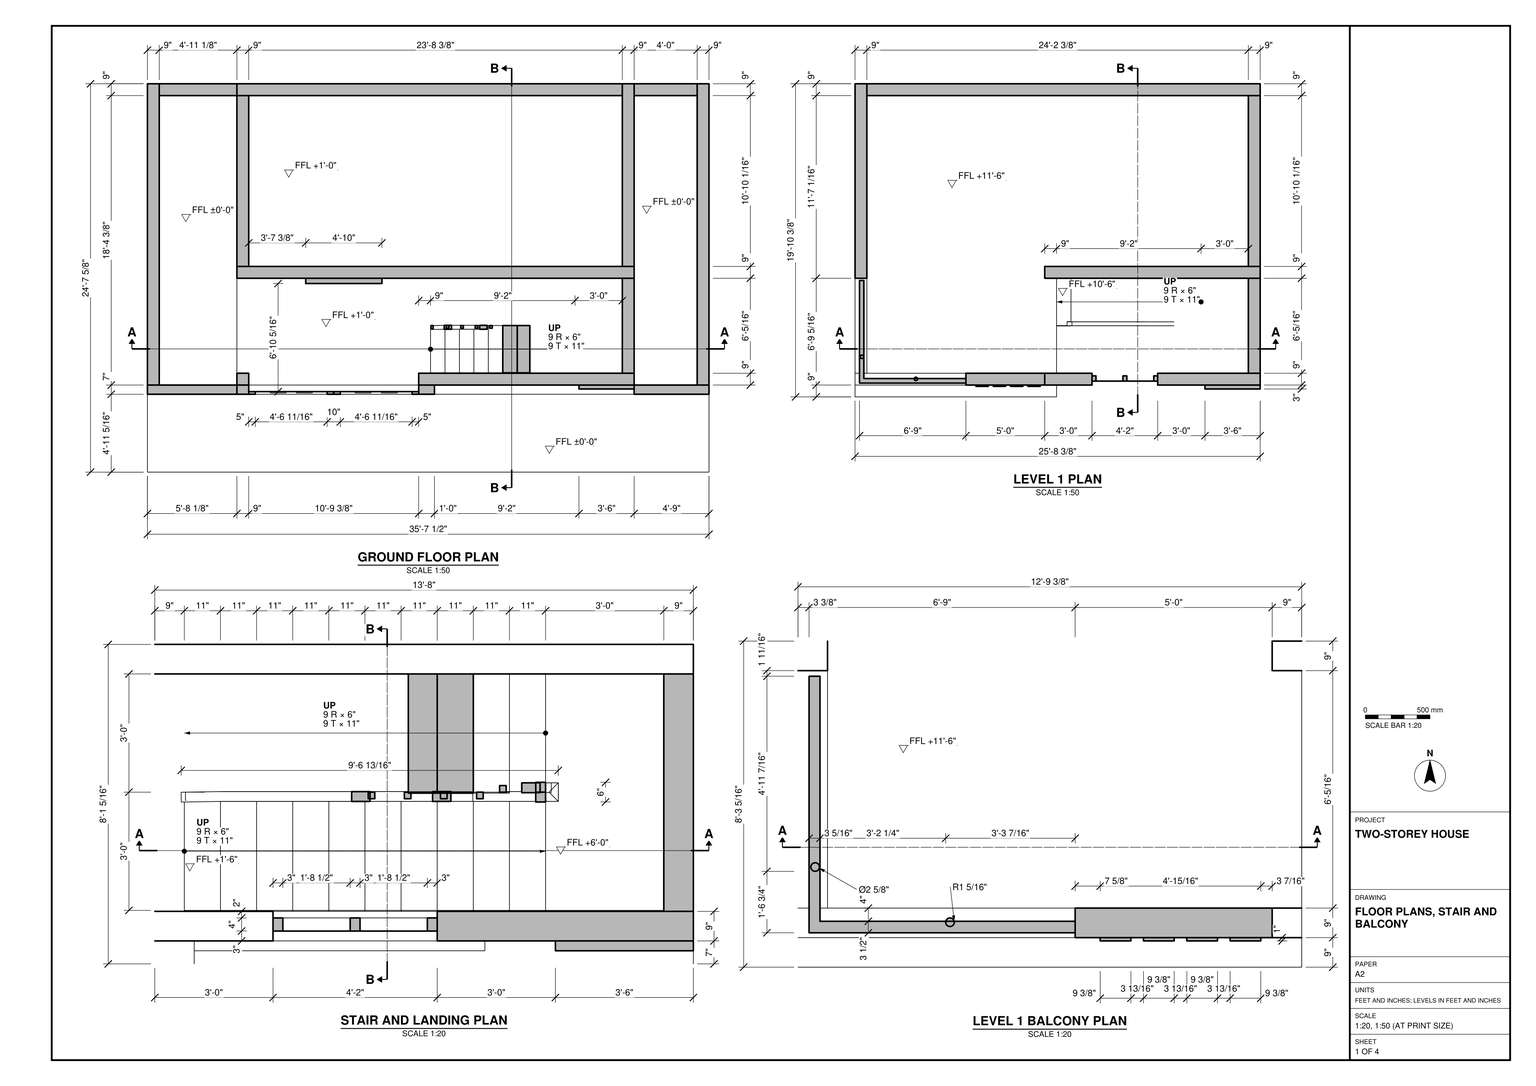
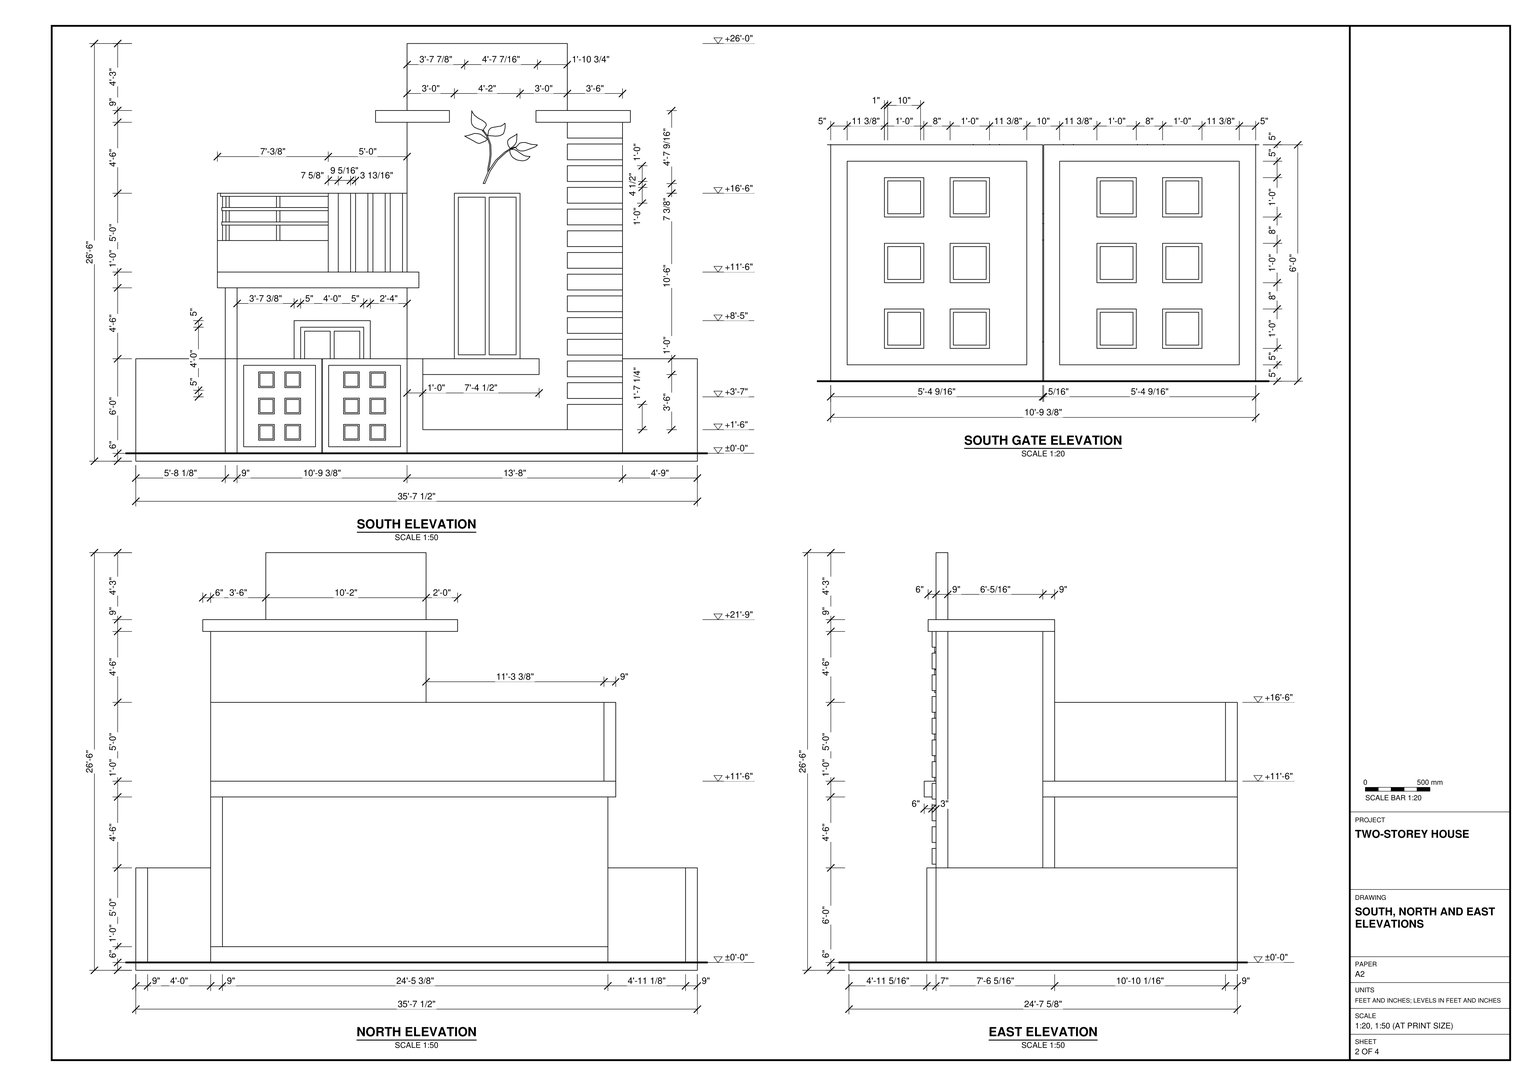
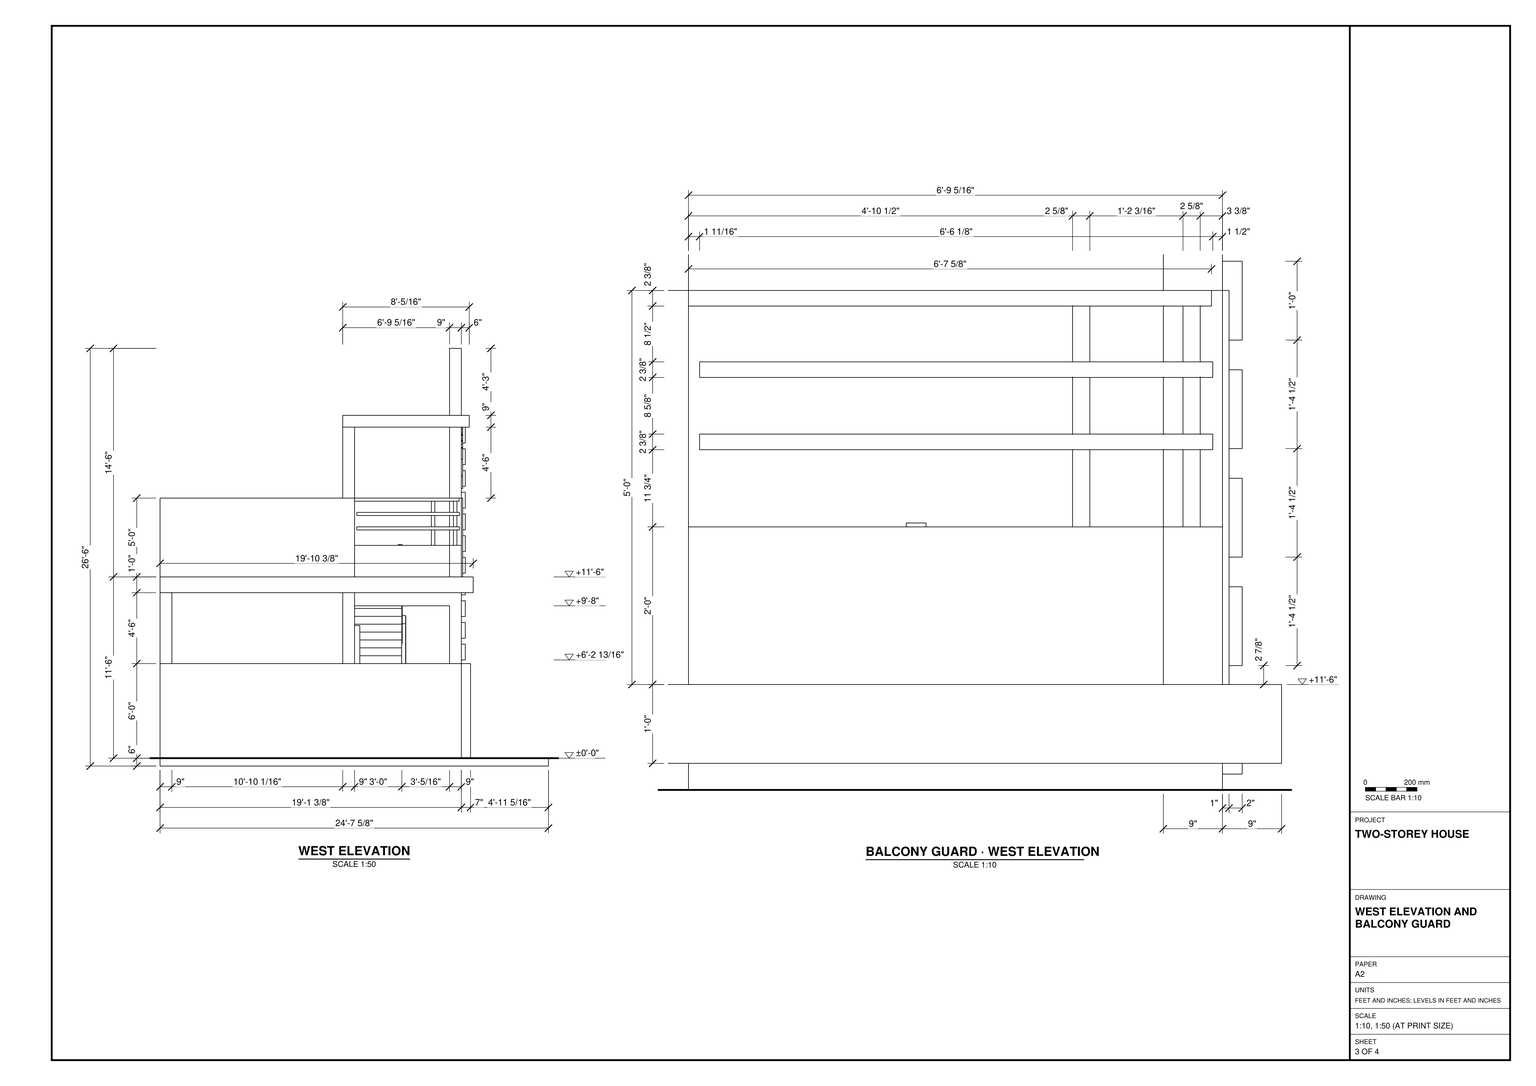
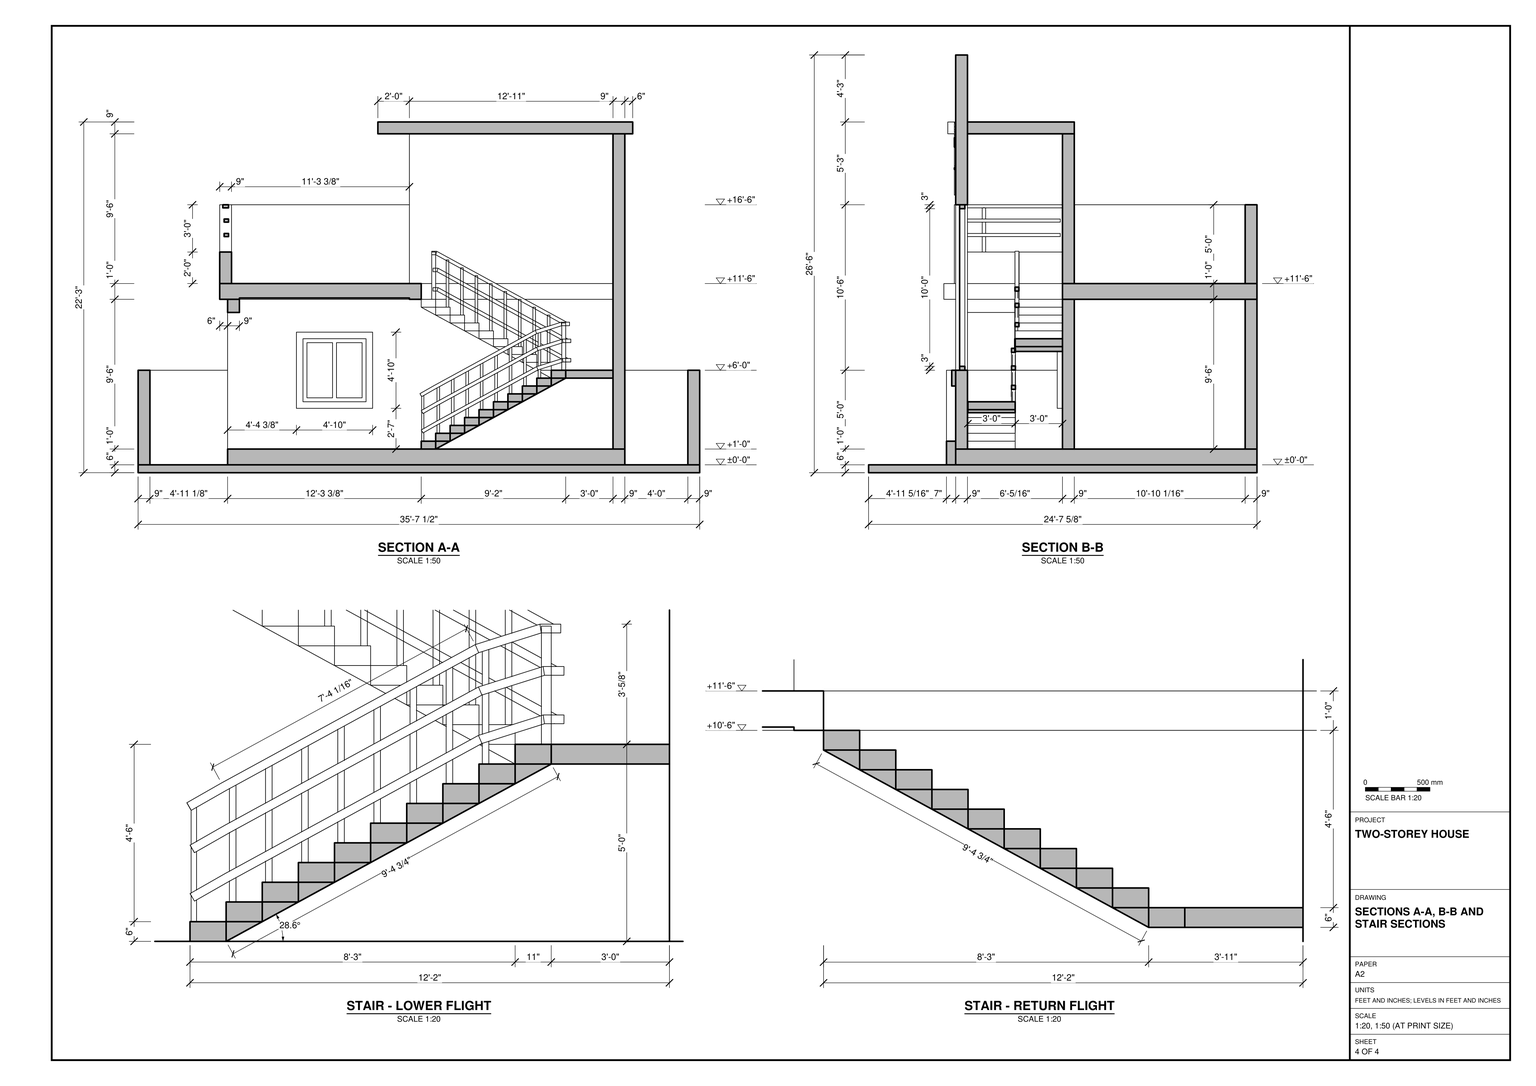
Build the two-storey house in SketchUp from task_files/diagram_01.pdf. Work in feet and inches. The overall model measures 35'-7 1/2" east to west, 24'-7 5/8" north to south and 26'-6" from the underside of the base to the highest wall. Use ±0'-0" as the ground-floor datum and +11'-6" as the Level 1 finished floor.

Start with the base slab, leaving the apron in front of the south gate and the narrow strips to either side of the house. Follow the ground-floor plan for the raised central floor, wall positions and 9" wall thicknesses where indicated. Model the paired gate leaves with their inset square panels and the framed opening behind the gate. Build the stair as two parallel flights that reverse direction at a common landing. Coordinate the stair opening in the upper slab with the flights below.

Use the elevations to distinguish the low terrace walls and balcony guard from the taller stair enclosure. Include the balcony slab edge, horizontal rails, uprights and adjoining vertical screen. Model the tall paired opening, projecting sill and horizontal bands on the south face of the stair enclosure, with the flat roof and raised wall above it. Decor and loose items shown may be represented by any suitable library component.

Keep shell elements such as walls, slabs and roof separate as groups or components. Group each furniture or joinery piece separately where shown, and use components for repeated parts. Save one SketchUp model as output_files/two_storey_house_with_a_return_stair_and_balcony.skp.

# SketchUp Ruby script. Lengths in inches.
U = 1.inch
M = Sketchup.active_model
def pt(a) = Geom::Point3d.new(a.map { |v| v * U })
def face(e, loops, mat)
  f = e.add_face(loops[0].map { |a| pt(a) })
  loops[1..].each { |l| e.add_face(l.map { |a| pt(a) }).erase! }
  f.material = f.back_material = mat if mat
  f
end
# faces: each face lists its corners as indices into pts; further lists are holes
def faces(e, pts, list, mat = nil) = list.each { |f| face(e, (f[0].is_a?(Array) ? f : [f]).map { |l| l.map { |i| pts[i] } }, mat) }
# xy, xz, yz: faces in a plane at the given z, y or x. An outline is a flat list of corners, or four numbers for a rectangle; further outlines are holes
def ring(l) = l.size == 4 ? [[l[0], l[1]], [l[2], l[1]], [l[2], l[3]], [l[0], l[3]]] : l.each_slice(2).to_a
def flat(e, list, mat, &to3) = list.each { |f| face(e, (f[0].is_a?(Array) ? f : [f]).map { |l| ring(l).map { |u, v| to3.(u, v) } }, mat) }
def xy(e, z, list, mat = nil) = flat(e, list, mat) { |x, y| [x, y, z] }
def xz(e, y, list, mat = nil) = flat(e, list, mat) { |x, z| [x, y, z] }
def yz(e, x, list, mat = nil) = flat(e, list, mat) { |y, z| [x, y, z] }
def lines(e, pts, list) = list.each { |a, b| e.add_line(pt(pts[a]), pt(pts[b])) }
# prism: a flat outline (further loops are holes) pulled along v
def prism(e, loops, v, mat = nil)
  f = face(e, loops, mat); d = Geom::Vector3d.new(v.map { |x| x * U })
  f.pushpull(f.normal.samedirection?(d) ? d.length : -d.length)
end
def box(e, o, s, mat = nil) = prism(e, [[o, [o[0] + s[0], o[1], o[2]], [o[0] + s[0], o[1] + s[1], o[2]], [o[0], o[1] + s[1], o[2]]]], [0, 0, s[2]], mat)
def at(x, y, z, deg = 0) = Geom::Transformation.translation(pt([x, y, z])) * Geom::Transformation.rotation(ORIGIN, Z_AXIS, deg.degrees)
def axes(o, x, y, z) = Geom::Transformation.new([*x, 0, *y, 0, *z, 0, *pt(o).to_a, 1])
def part(name) = M.definitions.add(name)
# library, detail: a bought-in or finely detailed component or shape, given as its bounding box
def library(name, o, s) = part(name).tap { |d| box(d.entities, o, s) }
def detail(e, o, s) = box(e.add_group.entities, o, s)
def put(e, d, t, mat = nil) = e.add_instance(d, t).tap { |i| i.material = mat if mat }
def group(e, t, mat = nil) = e.add_group.tap { |g| g.transformation = t; g.material = mat if mat }.entities
root = M.entities
M.materials.add("[Color M05]").color = [114, 114, 114]
M.materials.add("[Color M07]").color = [58, 58, 58]
M.materials.add("[Color M08]").color = [30, 30, 30]
M.materials.add("[Color M09]").color = [0, 0, 0]
M.materials.add("[Translucent Glass Gray]").color = [128, 128, 128]
M.materials["[Translucent Glass Gray]"].alpha = 0.5
c1 = part("Group\#4")
box(c1.entities,[0,0,0],[11,36,6])
c2 = part("Group\#5")
put(c2.entities,c1,at(22,0,12))
put(c2.entities,c1,at(11,0,6))
put(c2.entities,c1,at(44,0,24))
put(c2.entities,c1,at(33,0,18))
put(c2.entities,c1,at(0,0,0))
put(c2.entities,c1,at(55,0,30))
put(c2.entities,c1,at(99,0,54))
put(c2.entities,c1,at(66,0,36))
put(c2.entities,c1,at(77,0,42))
put(c2.entities,c1,at(88,0,48))
c3 = part("Group\#29")
box(c3.entities,[0,0,0],[3,3,36])
c4 = part("Group\#30")
xy(c4.entities,54.043,[[111.041,3.014,111.041,3.017,111.043,3.016]])
xy(c4.entities,56.716,[[111.723,3.695,113.885,5.858,111.723,5.858]])
yz(c4.entities,8.98,[[2.837,108.043,2.858,110.715,5.858,110.716,5.836,108.044]])
p = [[1.324,3.021,0],[1.361,0.022,0.021],[0.037,0,2.343],[0,2.999,2.321],[11.872,0.195,6.018],[10.57,0.173,8.352],
  [11.853,3.195,6.007],[10.552,3.173,8.341],[77.866,0.195,42.014],[88.886,0.195,48.025],[87.834,0.173,50.496],[76.586,0.173,44.36],
  [65.586,0.173,38.36],[54.586,0.173,32.36],[43.586,0.173,26.36],[32.586,0.173,20.36],[21.586,0.173,14.36],[22.866,0.195,12.014],
  [33.866,0.195,18.014],[44.866,0.195,24.014],[55.866,0.195,30.014],[66.866,0.195,36.014],[77.866,3.195,42.014],[88.886,3.195,48.025],
  [22.866,3.195,12.014],[33.866,3.195,18.014],[44.866,3.195,24.014],[55.866,3.195,30.014],[66.866,3.195,36.014],[76.586,3.173,44.36],
  [87.834,3.173,50.495],[21.586,3.173,14.36],[32.586,3.173,20.36],[43.586,3.173,26.36],[54.586,3.173,32.36],[65.586,3.173,38.36],
  [107.944,0.195,54.044],[107.532,0.173,56.716],[107.944,3.195,54.043],[107.532,3.173,56.715],[113.864,0.195,54.044],[113.885,0.173,56.716],
  [110.864,3.195,54.043],[111.041,3.017,54.043],[111.043,3.016,54.043],[113.864,5.836,54.044],[113.885,5.858,56.716],[100.095,2.837,60.014],
  [89.095,2.837,66.014],[78.095,2.837,72.014],[67.095,2.837,78.014],[56.095,2.837,84.014],[45.095,2.837,90.014],[34.095,2.837,96.014],
  [23.095,2.837,102.014],[12.041,2.837,108.043],[12.042,5.836,108.044],[23.095,5.836,102.014],[34.095,5.836,96.014],[45.095,5.836,90.014],
  [56.095,5.836,84.014],[67.095,5.836,78.014],[78.095,5.836,72.014],[89.095,5.836,66.014],[100.095,5.836,60.014],[111.042,5.836,54.044],
  [111.041,3.014,54.043],[111.041,2.837,54.043],[35.375,2.858,98.36],[24.375,2.858,104.36],[12.723,2.858,110.715],[111.723,2.858,56.715],
  [101.375,2.858,62.36],[90.375,2.858,68.36],[79.375,2.858,74.36],[68.375,2.858,80.36],[57.375,2.858,86.36],[46.375,2.858,92.36],
  [110.885,3.173,56.715],[12.723,5.858,110.716],[24.375,5.858,104.36],[35.375,5.858,98.36],[46.375,5.858,92.36],[57.375,5.858,86.36],
  [68.375,5.858,80.36],[79.375,5.858,74.36],[90.375,5.858,68.36],[101.375,5.858,62.36],[111.723,5.858,56.716],[111.043,3.016,56.715],
  [111.723,3.695,56.716],[8.98,2.837,108.043],[8.98,5.836,108.044],[8.98,2.858,110.715],[8.98,5.858,110.716]]
faces(c4.entities,p,[[0,1,2,3],[2,1,4,5],[1,0,6,4],[0,3,7,6],[3,2,5,7],[8,9,10,11,12,13,14,15,16,5,4,17,18,19,20,21],[22,23,9,8,21,20,19,18,17,4,6,24,25,26,27,28],[29,30,23,22,28,27,26,25,24,6,7,31,32,33,34,35],
  [11,10,30,29,35,34,33,32,31,7,5,16,15,14,13,12],[10,9,36,37],[9,23,38,36],[23,30,39,38],[30,10,37,39],[37,36,40,41],[36,38,42,43,44,40],[45,40,44],
  [41,40,45,46],[47,48,49,50,51,52,53,54,55,56,57,58,59,60,61,62,63,64,65,43,66,67],[68,69,70,55,54,53,52,51,50,49,48,47,67,71,72,73,74,75,76,77],[45,44,43,65],[38,39,78,42],[61,60,59,58,57,56,79,80,81,82,83,84,85,86,87,88,65,64,63,62],[46,45,65,88],[39,37,41,89,78],
  [41,46,90,89],[71,90,88,87,86,85,84,83,82,81,80,79,70,69,68,77,76,75,74,73,72],[56,55,91,92],[55,70,93,91],[79,56,92,94],[70,79,94,93]])
c5 = part("Group\#49")
box(c5.entities,[0,0,0],[42,3,12])
c6 = part("Group\#52")
box(c6.entities,[0,0,0],[9.34,1,60])
c7 = part("Group\#55")
prism(c7.entities,[[[82.03,5,0],[82.03,1.5,0],[1,1.5,0],[1,79.63,0],[4.34,79.63,0],[4.34,5,0]]],[0,0,2.375])
c8 = part("Group\#57")
prism(c8.entities,[[[0.38,2.24,0],[0.66,2.45,0],[0.97,2.58,0],[1.3125,2.625,0],[1.65,2.58,0],[1.97,2.45,0],[2.24,2.24,0],[2.45,1.97,0],[2.58,1.65,0],[2.625,1.3125,0],[2.58,0.97,0],[2.45,0.66,0],[2.24,0.38,0],[1.97,0.18,0],[1.65,0.04,0],[1.3125,0,0],[0.97,0.04,0],[0.66,0.18,0],[0.38,0.38,0],[0.18,0.66,0],[0.04,0.97,0],[0,1.3125,0],[0.04,1.65,0],[0.18,1.97,0]]],[0,0,33.75])
c9 = part("Group\#62")
prism(c9.entities,[[[12,0,0],[12,0,12],[0,0,12],[0,0,0]],[[11,0,11],[11,0,1],[1,0,1],[1,0,11]]],[0,1,0])
p = [[216,109.92,60],[226.51,110.09,66],[237.51,110.09,72],[248.51,110.09,78],[259.51,110.09,84],[270.51,110.09,90],
  [281.51,110.09,96],[292.51,110.09,102],[303.51,110.09,108],[322.51,110.09,114],[327.08,110.09,114],[327.08,113.09,114],
  [325.51,113.09,114],[314.51,113.09,120],[303.51,113.09,126],[292.51,113.09,132],[281.51,113.09,138],[270.51,113.09,144],
  [259.51,113.09,150],[248.51,113.09,156],[237.51,113.09,162],[226.51,113.09,168],[223.51,113.09,168],[215.51,66.29,132],
  [215.51,66.29,144],[206.51,66.29,132],[206.51,66.29,258],[238.78,66.29,258],[238.78,66.29,267],[206.51,66.29,267],
  [328.51,66.29,267],[304.64,66.29,267],[304.64,66.29,258],[328.51,66.29,258]]
lines(root,p,[[0,1],[1,2],[2,3],[3,4],[4,5],[5,6],[6,7],[7,8],[8,9],[9,10],[10,11],[11,12],
  [12,13],[13,14],[14,15],[15,16],[16,17],[17,18],[18,19],[19,20],[20,21],[21,22],[23,24],[25,23],
  [26,27],[27,28],[29,28],[30,31],[31,32],[32,33]])
g1 = group(root,at(84,0,0))
box(g1,[-84,0,0],[427.5,295.66,6])
g2 = group(root,at(128.11,75.59,6))
box(g2,[-60,-9.3,0],[302.4,229.36,12])
g3 = group(root,at(128.11,147.59,18))
prism(g3,[[[-60,0,0],[242.4,0,0],[242.4,0,114],[-60,0,114]],[[-2.6,0,84],[45.4,0,84],[45.4,0,36],[-2.6,0,36]]],[0,9,0])
put(root,c2,at(215.51,75.59,18))
g4 = group(root,at(325.51,75.59,72))
box(g4,[0,0,0],[36,72,6])
put(root,c2,at(325.51,147.59,72,-180))
g5 = group(root,at(215.51,111.59,72))
xy(g5,6,[[88,0,99,36]])
xy(g5,12,[[77,0,88,36]])
xy(g5,18,[[66,0,77,36]])
xy(g5,24,[[55,0,66,36]])
xy(g5,30,[[44,0,55,36]])
xy(g5,36,[[33,0,44,36]])
xy(g5,42,[[22,0,33,36]])
xy(g5,48,[[11,0,22,36]])
xy(g5,54,[[0,0,11,36]])
xz(g5,0,[[99,0,99,6,88,6],[88,6,88,12,77,12],[77,12,77,18,66,18],[66,18,66,24,55,24],[55,24,55,30,44,30],
  [44,30,44,36,33,36],[33,36,33,42,22,42],[22,42,22,48,11,48],[11,48,11,54,0,54]])
xz(g5,36,[[99,0,88,6,99,6],[88,6,77,12,88,12],[77,12,66,18,77,18],[66,18,55,24,66,24],[55,24,44,30,55,30],
  [44,30,33,36,44,36],[33,36,22,42,33,42],[22,42,11,48,22,48],[11,48,0,54,11,54]])
yz(g5,11,[[0,48,36,54]])
yz(g5,22,[[0,42,36,48]])
yz(g5,33,[[0,36,36,42]])
yz(g5,44,[[0,30,36,36]])
yz(g5,55,[[0,24,36,30]])
yz(g5,66,[[0,18,36,24]])
yz(g5,77,[[0,12,36,18]])
yz(g5,88,[[0,6,36,12]])
yz(g5,99,[[0,0,36,6]])
p = [[99,0,0],[88,0,6],[88,36,6],[99,36,0],[77,0,12],[77,36,12],
  [66,0,18],[66,36,18],[55,0,24],[55,36,24],[44,0,30],[44,36,30],
  [33,0,36],[33,36,36],[22,0,42],[22,36,42],[11,0,48],[11,36,48],
  [0,0,54],[0,36,54]]
faces(g5,p,[[0,1,2,3],[1,4,5,2],[4,6,7,5],[6,8,9,7],[8,10,11,9],[10,12,13,11],[12,14,15,13],[14,16,17,15],
  [16,18,19,17]])
g6 = group(root,at(226.51,75.59,18))
xy(g6,6,[[0,0,11,36]])
xy(g6,12,[[11,0,22,36]])
xy(g6,18,[[22,0,33,36]])
xy(g6,24,[[33,0,44,36]])
xy(g6,30,[[44,0,55,36]])
xy(g6,36,[[55,0,66,36]])
xy(g6,42,[[66,0,77,36]])
xy(g6,48,[[77,0,88,36]])
xy(g6,54,[[88,0,99,36]])
xz(g6,0,[[0,0,11,6,0,6],[11,6,22,12,11,12],[22,12,33,18,22,18],[33,18,44,24,33,24],[44,24,55,30,44,30],
  [55,30,66,36,55,36],[66,36,77,42,66,42],[77,42,88,48,77,48],[88,48,99,54,88,54]])
xz(g6,36,[[0,0,0,6,11,6],[11,6,11,12,22,12],[22,12,22,18,33,18],[33,18,33,24,44,24],[44,24,44,30,55,30],
  [55,30,55,36,66,36],[66,36,66,42,77,42],[77,42,77,48,88,48],[88,48,88,54,99,54]])
yz(g6,0,[[0,0,36,6]])
yz(g6,11,[[0,6,36,12]])
yz(g6,22,[[0,12,36,18]])
yz(g6,33,[[0,18,36,24]])
yz(g6,44,[[0,24,36,30]])
yz(g6,55,[[0,30,36,36]])
yz(g6,66,[[0,36,36,42]])
yz(g6,77,[[0,42,36,43.0625],[0,43.0625,36,48]])
yz(g6,88,[[0,48,36,54]])
p = [[0,36,0],[11,36,6],[11,0,6],[0,0,0],[22,36,12],[22,0,12],
  [33,36,18],[33,0,18],[44,36,24],[44,0,24],[55,36,30],[55,0,30],
  [66,36,36],[66,0,36],[77,36,42],[77,0,42],[88,36,48],[88,0,48],
  [99,36,54],[99,0,54]]
faces(g6,p,[[0,1,2,3],[1,4,5,2],[4,6,7,5],[6,8,9,7],[8,10,11,9],[10,12,13,11],[12,14,15,13],[14,16,17,15],
  [16,18,19,17]])
g7 = group(root,at(215.51,75.29,18))
prism(g7,[[[11,0,0],[110,0,54],[146,0,54],[146,0,60],[99,0,60],[99,0,54],[88,0,54],[88,0,48],[77,0,48],[77,0,42],[66,0,42],[66,0,36],[55,0,36],[55,0,30],[44,0,30],[44,0,24],[33,0,24],[33,0,18],[22,0,18],[22,0,12],[11,0,12],[11,0,6],[0,0,6],[0,0,0]]],[0,0.3,0])
g8 = group(root,at(215.51,111.29,72))
prism(g8,[[[0,0,54],[99,0,0],[99,0,12],[88,0,12],[88,0,18],[77,0,18],[77,0,24],[66,0,24],[66,0,30],[55,0,30],[55,0,36],[44,0,36],[44,0,42],[33,0,42],[33,0,48],[22,0,48],[22,0,54],[11,0,54],[11,0,60],[0,0,60]]],[0,0.3,0])
g9 = group(root,at(215.51,108.59,24),"[Color M09]")
box(g9,[0.34,0.5,0],[1.66,2.5,36.6875])
g10 = group(root,at(226.51,108.59,30),"[Color M09]")
box(g10,[1,1,0],[2,2,36])
g11 = group(root,at(237.51,108.59,36),"[Color M09]")
box(g11,[1,1,0],[2,2,36])
g12 = group(root,at(248.51,108.59,42),"[Color M09]")
box(g12,[1,1,0],[2,2,36])
g13 = group(root,at(259.51,108.59,48),"[Color M09]")
box(g13,[1,1,0],[2,2,36])
g14 = group(root,at(270.51,108.59,54),"[Color M09]")
box(g14,[1,1,0],[2,2,36])
g15 = group(root,at(281.51,108.59,60),"[Color M09]")
box(g15,[1,1,0],[2,2,36])
g16 = group(root,at(292.51,108.59,66),"[Color M09]")
box(g16,[1,1,0],[2,2,36])
g17 = group(root,at(303.51,108.59,72),"[Color M09]")
box(g17,[1,1,0],[2,2,36])
put(root,c3,at(322.51,108.59,78),"[Color M09]")
put(root,c3,at(322.51,111.59,78),"[Color M09]")
g18 = group(root,at(311.51,111.59,84),"[Color M09]")
box(g18,[0,0,0],[2,2,36])
g19 = group(root,at(300.51,111.59,90),"[Color M09]")
box(g19,[0,0,0],[2,2,36])
g20 = group(root,at(289.51,111.59,96),"[Color M09]")
box(g20,[0,0,0],[2,2,36])
g21 = group(root,at(278.51,111.59,102),"[Color M09]")
box(g21,[0,0,0],[2,2,36])
g22 = group(root,at(267.51,111.59,108),"[Color M09]")
box(g22,[0,0,0],[2,2,36])
g23 = group(root,at(256.51,111.59,114),"[Color M09]")
box(g23,[0,0,0],[2,2,36])
g24 = group(root,at(245.51,111.59,120),"[Color M09]")
box(g24,[0,0,0],[2,2,36])
g25 = group(root,at(234.51,111.59,126),"[Color M09]")
box(g25,[0,0,0],[2,2,36])
put(root,c3,at(223.51,111.59,132),"[Color M09]")
put(root,c4,at(214.53,108.58,57.88),"[Color M09]")
g26 = group(root,at(215.51,108.59,44.98),"[Color M09]")
xy(g26,54.043,[[111.041,3.014,111.041,3.017,111.043,3.016]])
xy(g26,56.716,[[111.723,3.695,113.885,5.858,111.723,5.858]])
yz(g26,8.98,[[2.837,108.043,2.858,110.715,5.858,110.716,5.836,108.044]])
p = [[1.324,3.021,0],[1.361,0.022,0.021],[0.037,0,2.343],[0,2.999,2.321],[11.872,0.195,6.018],[10.57,0.173,8.352],
  [11.853,3.195,6.007],[10.552,3.173,8.341],[77.866,0.195,42.014],[88.886,0.195,48.025],[87.834,0.173,50.496],[76.586,0.173,44.36],
  [65.586,0.173,38.36],[54.586,0.173,32.36],[43.586,0.173,26.36],[32.586,0.173,20.36],[21.586,0.173,14.36],[22.866,0.195,12.014],
  [33.866,0.195,18.014],[44.866,0.195,24.014],[55.866,0.195,30.014],[66.866,0.195,36.014],[77.866,3.195,42.014],[88.886,3.195,48.025],
  [22.866,3.195,12.014],[33.866,3.195,18.014],[44.866,3.195,24.014],[55.866,3.195,30.014],[66.866,3.195,36.014],[76.586,3.173,44.36],
  [87.834,3.173,50.495],[21.586,3.173,14.36],[32.586,3.173,20.36],[43.586,3.173,26.36],[54.586,3.173,32.36],[65.586,3.173,38.36],
  [107.944,0.195,54.044],[107.532,0.173,56.716],[107.944,3.195,54.043],[107.532,3.173,56.715],[113.864,0.195,54.044],[113.885,0.173,56.716],
  [110.864,3.195,54.043],[111.041,3.017,54.043],[111.043,3.016,54.043],[113.864,5.836,54.044],[113.885,5.858,56.716],[100.095,2.837,60.014],
  [89.095,2.837,66.014],[78.095,2.837,72.014],[67.095,2.837,78.014],[56.095,2.837,84.014],[45.095,2.837,90.014],[34.095,2.837,96.014],
  [23.095,2.837,102.014],[12.041,2.837,108.043],[12.042,5.836,108.044],[23.095,5.836,102.014],[34.095,5.836,96.014],[45.095,5.836,90.014],
  [56.095,5.836,84.014],[67.095,5.836,78.014],[78.095,5.836,72.014],[89.095,5.836,66.014],[100.095,5.836,60.014],[111.042,5.836,54.044],
  [111.041,3.014,54.043],[111.041,2.837,54.043],[35.375,2.858,98.36],[24.375,2.858,104.36],[12.723,2.858,110.715],[111.723,2.858,56.715],
  [101.375,2.858,62.36],[90.375,2.858,68.36],[79.375,2.858,74.36],[68.375,2.858,80.36],[57.375,2.858,86.36],[46.375,2.858,92.36],
  [110.885,3.173,56.715],[12.723,5.858,110.716],[24.375,5.858,104.36],[35.375,5.858,98.36],[46.375,5.858,92.36],[57.375,5.858,86.36],
  [68.375,5.858,80.36],[79.375,5.858,74.36],[90.375,5.858,68.36],[101.375,5.858,62.36],[111.723,5.858,56.716],[111.043,3.016,56.715],
  [111.723,3.695,56.716],[8.98,2.837,108.043],[8.98,5.836,108.044],[8.98,2.858,110.715],[8.98,5.858,110.716]]
faces(g26,p,[[0,1,2,3],[2,1,4,5],[1,0,6,4],[0,3,7,6],[3,2,5,7],[8,9,10,11,12,13,14,15,16,5,4,17,18,19,20,21],[22,23,9,8,21,20,19,18,17,4,6,24,25,26,27,28],[29,30,23,22,28,27,26,25,24,6,7,31,32,33,34,35],
  [11,10,30,29,35,34,33,32,31,7,5,16,15,14,13,12],[10,9,36,37],[9,23,38,36],[23,30,39,38],[30,10,37,39],[37,36,40,41],[36,38,42,43,44,40],[45,40,44],
  [41,40,45,46],[47,48,49,50,51,52,53,54,55,56,57,58,59,60,61,62,63,64,65,43,66,67],[68,69,70,55,54,53,52,51,50,49,48,47,67,71,72,73,74,75,76,77],[45,44,43,65],[38,39,78,42],[61,60,59,58,57,56,79,80,81,82,83,84,85,86,87,88,65,64,63,62],[46,45,65,88],[39,37,41,89,78],
  [41,46,90,89],[71,90,88,87,86,85,84,83,82,81,80,79,70,69,68,77,76,75,74,73,72],[56,55,91,92],[55,70,93,91],[79,56,92,94],[70,79,94,93]])
put(root,c4,at(215.51,108.59,30.23),"[Color M09]")
g27 = group(root,at(361.51,75.29,18))
box(g27,[0,0,0],[9,72.3,240])
g28 = group(root,at(120.51,143.59,49))
prism(g28,[[[58,0,0],[58,0,58],[0,0,58],[0,0,0]],[[53,0,5],[5,0,5],[5,0,53],[53,0,53]]],[0,4,0])
g29 = group(root,at(125.51,147.59,54),"[Color M09]")
prism(g29,[[[48,4,48],[48,4,0],[0,4,0],[0,4,48]],[[22.5,4,3],[22.5,4,45],[3,4,45],[3,4,3]],[[45,4,45],[25.5,4,45],[25.5,4,3],[45,4,3]]],[0,-4,0])
g30 = group(root,at(151.01,147.59,57),"[Translucent Glass Gray]")
xz(g30,0,[[0,0,19.5,42]])
g31 = group(root,at(128.51,147.59,57),"[Translucent Glass Gray]")
xz(g31,0,[[0,0,19.5,42]])
g32 = group(root,at(68.11,156.59,18))
box(g32,[0,0,0],[9,130.0625,114])
g33 = group(root,at(68.11,286.66,18))
box(g33,[0,0,0],[293.4,9,114])
g34 = group(root,at(361.51,156.59,18))
box(g34,[0,0,0],[9,139.0625,114])
g35 = group(root,at(68.11,147.59,132))
xy(g35,0,[[[-6,-90.3,-6,148.0625,302.4,148.0625,302.4,0,147.4,0,147.4,-90.3],[9,-72.3,138.4,0]]],"[Color M07]")
xy(g35,1,[[9,-72.3,138.4,0]])
xy(g35,12,[[-6,-90.3,147.4,-90.3,147.4,0,302.4,0,302.4,148.0625,-6,148.0625]])
xz(g35,-90.3,[[-6,0,147.4,12]],"[Color M07]")
xz(g35,-72.3,[[9,0,138.4,1]])
xz(g35,0,[[9,0,138.4,1],[147.4,0,302.4,12]])
xz(g35,148.0625,[[-6,0,302.4,12]])
yz(g35,-6,[[-90.3,0,148.0625,12]],"[Color M07]")
yz(g35,9,[[-72.3,0,0,1]])
yz(g35,138.4,[[-72.3,0,0,1]])
yz(g35,147.4,[[-90.3,0,0,12]],"[Color M07]")
yz(g35,302.4,[[0,0,148.0625,12]])
g36 = group(root,at(68.11,66.29,18))
prism(g36,[[[0,9,0],[0,0,0],[0,0,114],[0,81.3,114],[0,81.3,104],[0,9,104]]],[9,0,0])
g37 = group(root,at(242.51,69.29,78),"[Color M09]")
prism(g37,[[[50,4,126],[50,4,0],[0,4,0],[0,4,126]],[[23.5,4,3],[23.5,4,123],[3,4,123],[3,4,3]],[[47,4,123],[26.5,4,123],[26.5,4,3],[47,4,3]]],[0,-4,0])
g38 = group(root,at(269.01,69.29,81),"[Translucent Glass Gray]")
xz(g38,0,[[0,0,20.5,120]])
g39 = group(root,at(245.51,69.29,81),"[Translucent Glass Gray]")
xz(g39,0,[[0,0,20.5,120]])
g40 = group(root,at(206.51,147.59,144))
box(g40,[0,0,0],[164,9,114])
g41 = group(root,at(206.51,66.29,258),"[Color M07]")
prism(g41,[[[-24,-6,0],[-24,90.3,0],[170,90.3,0],[170,-6,0],[98.13,-6,0],[98.13,9,0],[32.26,9,0],[32.26,-6,0]]],[0,0,9])
g42 = group(root,at(206.51,63.29,6))
prism(g42,[[[164,3,18],[164,3,0],[0,3,0],[0,3,72],[12,3,72],[12,3,18]]],[0,-7,0])
put(root,c5,at(328.51,63.29,246),"[Color M07]")
put(root,c5,at(328.51,63.29,229.48),"[Color M07]")
put(root,c5,at(328.51,63.29,212.96),"[Color M07]")
put(root,c5,at(328.51,63.29,196.44),"[Color M07]")
put(root,c5,at(328.51,63.29,179.92),"[Color M07]")
put(root,c5,at(328.51,63.29,163.4),"[Color M07]")
put(root,c5,at(328.51,63.29,146.88),"[Color M07]")
put(root,c5,at(328.51,63.29,130.37),"[Color M07]")
put(root,c5,at(328.51,63.29,113.85),"[Color M07]")
put(root,c5,at(328.51,63.29,97.33),"[Color M07]")
put(root,c5,at(328.51,63.29,80.81),"[Color M07]")
put(root,c5,at(328.51,63.29,64.29),"[Color M07]")
put(root,c5,at(328.51,63.29,47.77),"[Color M07]")
g43 = group(root,at(328.51,63.29,31.25),"[Color M07]")
box(g43,[0,0,-7.25],[42,3,19.25])
g44 = group(root,at(146.51,66.29,144))
box(g44,[0,0,0],[60,9,60])
p = [[69,0,0],[60,0,0]]
lines(g44,p,[[0,1]])
g45 = group(root,at(62.11,66.29,144))
box(g45,[0,0,0],[84.4,9,24])
put(root,c6,at(193.71,65.29,144),"[Color M05]")
put(root,c6,at(180.52,65.29,144),"[Color M05]")
put(root,c6,at(167.33,65.29,144),"[Color M05]")
put(root,c6,at(154.14,65.29,144),"[Color M05]")
g46 = group(root,at(62.11,147.59,144))
box(g46,[0,0,0],[9,148.0625,60])
g47 = group(root,at(62.11,75.29,144))
box(g47,[0,0,0],[9,72.3,24])
g48 = group(root,at(64.49,67.96,201.625),"[Color M07]")
prism(g48,[[[82.03,5,0],[82.03,0,0],[0,0,0],[0,79.63,0],[4.34,79.63,0],[4.34,5,0]]],[0,0,2.375])
put(root,c7,at(64.49,66.27,190.76),"[Color M07]")
put(root,c7,at(64.49,66.27,179.76),"[Color M07]")
put(root,c8,at(107.09,69.68,168),"[Color M07]")
put(root,c8,at(66.03,86.49,168),"[Color M07]")
g49 = group(root,at(361.51,156.59,144))
box(g49,[0,0,0],[9,130.0625,60])
g50 = group(root,at(71.11,286.66,144))
box(g50,[0,0,0],[299.4,9,60])
g51 = group(root,at(68.11,59.29,6))
box(g51,[0,0,0],[9,7,72])
g52 = group(root,at(77.11,56.29,6),"[Color M07]")
xy(g52,0,[[0,3,64.55,5],[64.85,3,129.4,5]])
xy(g52,5,[[5,3,59.7,5],[69.7,3,124.4,5]])
xy(g52,67,[[5,3,59.7,5],[69.7,3,124.4,5]])
xy(g52,72,[[0,3,64.55,5],[64.85,3,129.4,5]])
xz(g52,3,[[[0,0,64.55,72],[5,5,59.7,67]],[[64.85,0,129.4,72],[69.7,5,124.4,67]]],"[Color M08]")
xz(g52,5,[[[0,0,64.55,72],[5,5,59.7,67]],[[64.85,0,129.4,72],[69.7,5,124.4,67]],[5,5,59.7,67],[69.7,5,124.4,67]])
yz(g52,0,[[3,0,5,72]])
yz(g52,5,[[3,5,5,67]])
yz(g52,59.7,[[3,5,5,67]])
yz(g52,64.55,[[3,0,5,72]])
yz(g52,64.85,[[3,0,5,72]])
yz(g52,69.7,[[3,5,5,67]])
yz(g52,124.4,[[3,5,5,67]])
yz(g52,129.4,[[3,0,5,72]])
put(root,c9,at(93.46,60.29,36),"[Color M08]")
put(root,c9,at(93.46,60.29,16),"[Color M08]")
put(root,c9,at(93.46,60.29,56),"[Color M08]")
put(root,c9,at(113.46,60.29,56),"[Color M08]")
put(root,c9,at(113.46,60.29,36),"[Color M08]")
put(root,c9,at(113.46,60.29,16),"[Color M08]")
put(root,c9,at(178.16,60.29,36),"[Color M08]")
put(root,c9,at(158.16,60.29,16),"[Color M08]")
put(root,c9,at(178.16,60.29,56),"[Color M08]")
put(root,c9,at(178.16,60.29,16),"[Color M08]")
put(root,c9,at(158.16,60.29,56),"[Color M08]")
put(root,c9,at(158.16,60.29,36),"[Color M08]")
g53 = group(root,at(218.51,63.29,66),"[Color M07]")
box(g53,[0,0,0],[88.52,3,12])
g54 = group(root,at(215.51,66.29,18))
prism(g54,[[[155,9,0],[-9,9,0],[-9,9,300],[113,9,300],[113,9,240],[155,9,240]],[[77,9,60],[77,9,186],[27,9,186],[27,9,60]]],[0,-9,0])
g55 = group(root,at(264.42,65.29,211.36),"[Color M07]")
prism(g55,[[[20.48,1,26.57],[20.48,1,26.6],[20.32,1,26.88],[19.97,1,27.52],[19.07,1,29.09],[18.58,1,31.01],[18.59,1,31.78],[18.87,1,32.86],[19.42,1,33.64],[20.09,1,34.26],[22.02,1,35.4],[25.36,1,37.38],[25.59,1,37.77],[25.67,1,37.93],[25.79,1,37.8125],[25.72,1,37.08],[25.6,1,35.29],[25.53,1,33.3],[25.3,1,31.61],[24.37,1,29.91],[23.2,1,28.6],[21.84,1,27.54],[21.2,1,27.15],[20.92,1,26.95]]],[0,-1,0])
xy(g55,0,[[0,0,1.3125,1]])
xy(g55,27.73,[[23.74,0,25.05,1]])
xz(g55,0,[[0,0,1.3125,0,5.32,9.47,10.99,17.88,17.71,23.96,20.4,25.64,20.51,25.71,21.07,26.06,24.63,27.55,25.05,27.73,23.74,27.73,20.92,26.55,20.5,26.37,20.35,26.31,19.75,26.06,16.4,23.96,9.68,17.88,4,9.47],[29.63,17.35,30.88,17.4,32.46,17.8,33.65,18.43,34.69,19.36,35.49,20.375,35.66,20.64,35.7,20.76,35.57,20.68,34.88,20.62,33.57,20.79,31.83,21.09,30.48,21.71,28.01,23.32,26.1,24.71,24.25,25.78,23.3125,25.9375,22.47,25.99,21.07,26.06,20.51,25.71,20.41,25.52,20.4,25.31,20.38,25.03,20.35,24.29,20.5,23.49,20.73,22.75,21.5625,21.12,22.21,20.25,23.06,19.55,25.24,18.23,26.28,17.88,27.65,17.6],[28.48,24.8,30.79,24.875,32.47,25.27,37.64,27.19,39.97,28.21,41.35,29.45,36.5625,29.9,32.24,31.27,29.83,31.28,27.75,30.78,25.05,27.73,24.63,27.55,25.57,26.28,26.4,25.65]])
xz(g55,1,[[0,0,4,9.47,9.68,17.88,16.4,23.96,19.75,26.06,20.35,26.31,20.5,26.37,20.92,26.55,23.74,27.73,25.05,27.73,24.63,27.55,21.07,26.06,20.51,25.71,20.4,25.64,17.71,23.96,10.99,17.88,5.32,9.47,1.3125,0]])
p = [[4,1,9.47],[0,1,0],[0,0,0],[4,0,9.47],[1.3125,1,0],[5.32,1,9.47],
  [5.32,0,9.47],[1.3125,0,0],[9.68,1,17.88],[9.68,0,17.88],[10.99,1,17.88],[10.99,0,17.88],
  [27.65,1,17.6],[29.63,1,17.35],[29.63,0,17.35],[27.65,0,17.6],[30.88,1,17.4],[30.88,0,17.4],
  [32.46,1,17.8],[32.46,0,17.8],[26.28,1,17.88],[26.28,0,17.88],[33.65,1,18.43],[33.65,0,18.43],
  [16.4,1,23.96],[16.4,0,23.96],[17.71,1,23.96],[17.71,0,23.96],[25.24,1,18.23],[25.24,0,18.23],
  [23.06,1,19.55],[23.06,0,19.55],[34.69,1,19.36],[34.69,0,19.36],[35.49,1,20.375],[35.49,0,20.375],
  [22.21,1,20.25],[22.21,0,20.25],[21.5625,1,21.12],[21.5625,0,21.12],[35.66,1,20.64],[35.66,0,20.64],
  [34.88,1,20.62],[33.57,1,20.79],[33.57,0,20.79],[34.88,0,20.62],[35.57,1,20.68],[35.57,0,20.68],
  [35.7,1,20.76],[35.7,0,20.76],[31.83,1,21.09],[31.83,0,21.09],[20.73,1,22.75],[20.73,0,22.75],
  [30.48,1,21.71],[30.48,0,21.71],[28.01,1,23.32],[28.01,0,23.32],[20.5,1,23.49],[20.5,0,23.49],
  [26.1,1,24.71],[26.1,0,24.71],[20.35,1,24.29],[20.35,0,24.29],[19.75,1,26.06],[19.75,0,26.06],
  [20.4,1,25.64],[20.4,0,25.64],[20.38,1,25.03],[20.38,0,25.03],[24.25,1,25.78],[24.25,0,25.78],
  [26.4,1,25.65],[28.48,1,24.8],[28.48,0,24.8],[26.4,0,25.65],[30.79,1,24.875],[30.79,0,24.875],
  [32.47,1,25.27],[32.47,0,25.27],[20.4,1,25.31],[20.4,0,25.31],[20.41,1,25.52],[20.41,0,25.52],
  [37.64,1,27.19],[37.64,0,27.19],[20.51,1,25.71],[20.51,0,25.71],[25.57,1,26.28],[25.57,0,26.28],
  [23.3125,1,25.9375],[23.3125,0,25.9375],[22.47,1,25.99],[22.47,0,25.99],[21.07,1,26.06],[21.07,0,26.06],
  [20.35,1,26.31],[20.35,0,26.31],[24.63,1,27.55],[24.63,0,27.55],[20.5,1,26.37],[20.5,0,26.37],
  [20.92,1,26.55],[20.92,0,26.55],[23.74,1,27.73],[23.74,0,27.73],[39.97,1,28.21],[39.97,0,28.21],
  [27.75,1,30.78],[25.05,1,27.73],[25.05,0,27.73],[27.75,0,30.78],[41.35,1,29.45],[41.35,0,29.45],
  [36.5625,1,29.9],[36.5625,0,29.9],[32.24,1,31.27],[32.24,0,31.27],[29.83,1,31.28],[29.83,0,31.28],
  [20.48,1,26.57]]
faces(g55,p,[[0,1,2,3],[4,5,6,7],[8,0,3,9],[5,10,11,6],[12,13,14,15],[13,16,17,14],[16,18,19,17],[20,12,15,21],
  [18,22,23,19],[24,8,9,25],[10,26,27,11],[28,20,21,29],[30,28,29,31],[22,32,33,23],[32,34,35,33],[36,30,31,37],
  [38,36,37,39],[34,40,41,35],[42,43,44,45],[46,42,45,47],[40,48,49,41],[48,46,47,49],[43,50,51,44],[52,38,39,53],
  [50,54,55,51],[54,56,57,55],[58,52,53,59],[56,60,61,57],[62,58,59,63],[64,24,25,65],[26,66,67,27],[68,62,63,69],
  [60,70,71,61],[72,73,74,75],[73,76,77,74],[76,78,79,77],[80,68,69,81],[82,80,81,83],[78,84,85,79],[86,82,83,87],
  [66,86,87,67],[88,72,75,89],[70,90,91,71],[90,92,93,91],[92,94,95,93],[96,64,65,97],[94,98,99,95],[100,96,97,101],
  [98,88,89,99],[102,100,101,103],[104,102,103,105],[84,106,107,85],[108,109,110,111],[106,112,113,107],[112,114,115,113],[114,116,117,115],
  [118,108,111,119],[116,118,119,117]])
lines(g55,p,[[120,96]])
g56 = group(root,at(250.36,65.29,220.21),"[Color M07]")
xy(g56,31.63,[[13.53,0,13.96,1]])
xz(g56,0,[[17.8,0,17.59,1.21,17.54,2.1,17.91,4.15,18.69,8.1,19.28,13.42,19.12,18.27,19.05,20.54,18.33,22.8,17.45,25.01,17.34,25.28,16.35,27.77,13.8,31.25,13.96,31.63,14.4,31.63,17.23,27.77,19.2,22.8,19.93,20.54,19.99,18.27,20.16,13.42,19.57,8.1,18.79,4.15,18.42,2.1,18.46,1.21,18.07,0.63],[11.21,21.67,9.875,21.99,8.97,22.37,4.53,24.87,0.65,26.9,0,27.38,0.38,27.39,1.2,27.46,3.5625,28.0625,7.54,29.37,9.96,29.14,11.1875,28.94,12.36,28.52,14.98,26.7,16.15,25.78,16.67,25.48,17.34,25.28,17.45,25.01,16.44,24.17,16.17,23.72,16.01,23.5,15.8,23.52,13.4,22.55],[23.47,27.23,24.53,27.36,26.5,27.54,28.89,28.6,29.61,29.35,30.06,30.61,30.77,33.51,30.83,35.85,30.77,36.7,30.66,37.17,30.46,36.96,29.34,36,28.21,35.18,27.27,34.89,22.05,34.03,20.68,33.78,19.46,33.13,18.31,31.59,17.79,29.23,17.79,28.41,17.23,27.77,22.04,27.4],[13.53,31.63,14.4,31.63,14.29,32.2,14.95,33.3,16.33,35.24,16.41,36.52,15.8,37.47,13.36,39.32,10.45,40.88,7.41,43.18,5.62,45.96,5.36,46.7,5.42,45.91,5.08,40.67,5.09,38.16,5.33,36.89,5.79,35.875,7.3125,34.125,9.53,33.04,11.95,32.22,13.15,32.01,13.43,31.98]])
xz(g56,1,[[23.47,27.23,22.04,27.4,17.23,27.77,17.79,28.41,17.79,29.23,18.31,31.59,19.46,33.13,20.68,33.78,22.05,34.03,27.27,34.89,28.21,35.18,29.34,36,30.46,36.96,30.66,37.17,30.77,36.7,30.83,35.85,30.77,33.51,30.06,30.61,29.61,29.35,28.89,28.6,26.5,27.54,24.53,27.36],[13.69,31,13.53,31.63,13.8,31.25],[13.8,31.25,13.53,31.63,13.96,31.63],[13.53,31.63,13.43,31.98,13.15,32.01,11.95,32.22,9.53,33.04,7.3125,34.125,5.79,35.875,5.33,36.89,5.09,38.16,5.08,40.67,5.42,45.91,5.36,46.7,5.62,45.96,7.41,43.18,10.45,40.88,13.36,39.32,15.8,37.47,16.41,36.52,16.33,35.24,14.95,33.3,14.29,32.2,14.4,31.63]])
yz(g56,17.79,[[0,28.41,1,29.23]])
p = [[17.8,1,0],[17.59,1,1.21],[17.59,0,1.21],[17.8,0,0],[18.07,1,0.63],[18.07,0,0.63],
  [18.46,1,1.21],[18.46,0,1.21],[17.54,1,2.1],[17.54,0,2.1],[18.42,1,2.1],[18.42,0,2.1],
  [17.91,1,4.15],[17.91,0,4.15],[18.79,1,4.15],[18.79,0,4.15],[18.69,1,8.1],[18.69,0,8.1],
  [19.57,1,8.1],[19.57,0,8.1],[19.28,1,13.42],[19.28,0,13.42],[20.16,1,13.42],[20.16,0,13.42],
  [19.12,1,18.27],[19.12,0,18.27],[19.99,1,18.27],[19.99,0,18.27],[19.05,1,20.54],[19.05,0,20.54],
  [19.93,1,20.54],[19.93,0,20.54],[18.33,1,22.8],[18.33,0,22.8],[19.2,1,22.8],[19.2,0,22.8],
  [11.21,1,21.67],[9.875,1,21.99],[9.875,0,21.99],[11.21,0,21.67],[13.4,1,22.55],[13.4,0,22.55],
  [8.97,1,22.37],[8.97,0,22.37],[4.53,1,24.87],[4.53,0,24.87],[15.8,1,23.52],[15.8,0,23.52],
  [17.23,1,27.77],[17.23,0,27.77],[17.45,1,25.01],[17.45,0,25.01],[16.01,1,23.5],[16.01,0,23.5],
  [16.17,1,23.72],[16.17,0,23.72],[16.44,1,24.17],[16.44,0,24.17],[0.65,1,26.9],[0.65,0,26.9],
  [17.34,1,25.28],[16.35,1,27.77],[16.35,0,27.77],[17.34,0,25.28],[16.67,1,25.48],[16.67,0,25.48],
  [16.15,1,25.78],[16.15,0,25.78],[14.98,1,26.7],[14.98,0,26.7],[12.36,1,28.52],[12.36,0,28.52],
  [0,1,27.38],[0,0,27.38],[22.04,1,27.4],[23.47,1,27.23],[23.47,0,27.23],[22.04,0,27.4],
  [24.53,1,27.36],[24.53,0,27.36],[0.38,1,27.39],[0.38,0,27.39],[1.2,1,27.46],[1.2,0,27.46],
  [26.5,1,27.54],[26.5,0,27.54],[3.5625,1,28.0625],[3.5625,0,28.0625],[28.89,1,28.6],[28.89,0,28.6],
  [13.8,1,31.25],[13.8,0,31.25],[14.4,1,31.63],[14.4,0,31.63],[17.79,1,28.41],[17.79,0,28.41],
  [7.54,1,29.37],[7.54,0,29.37],[11.1875,1,28.94],[11.1875,0,28.94],[29.61,1,29.35],[29.61,0,29.35],
  [9.96,1,29.14],[9.96,0,29.14],[18.31,1,31.59],[17.79,1,29.23],[17.79,0,29.23],[18.31,0,31.59],
  [30.06,1,30.61],[30.06,0,30.61],[30.77,1,33.51],[30.77,0,33.51],[13.96,1,31.63],[13.96,0,31.63],
  [13.43,1,31.98],[13.53,1,31.63],[13.53,0,31.63],[13.43,0,31.98],[14.29,1,32.2],[14.29,0,32.2],
  [19.46,1,33.13],[19.46,0,33.13],[11.95,1,32.22],[13.15,1,32.01],[13.15,0,32.01],[11.95,0,32.22],
  [9.53,1,33.04],[9.53,0,33.04],[14.95,1,33.3],[14.95,0,33.3],[7.3125,1,34.125],[7.3125,0,34.125],
  [20.68,1,33.78],[20.68,0,33.78],[16.33,1,35.24],[16.33,0,35.24],[30.83,1,35.85],[30.83,0,35.85],
  [22.05,1,34.03],[22.05,0,34.03],[27.27,1,34.89],[27.27,0,34.89],[5.79,1,35.875],[5.79,0,35.875],
  [28.21,1,35.18],[28.21,0,35.18],[16.41,1,36.52],[16.41,0,36.52],[29.34,1,36],[29.34,0,36],
  [5.33,1,36.89],[5.33,0,36.89],[30.77,1,36.7],[30.77,0,36.7],[30.46,1,36.96],[30.46,0,36.96],
  [15.8,1,37.47],[15.8,0,37.47],[30.66,1,37.17],[30.66,0,37.17],[5.09,1,38.16],[5.09,0,38.16],
  [13.36,1,39.32],[13.36,0,39.32],[5.08,1,40.67],[5.08,0,40.67],[10.45,1,40.88],[10.45,0,40.88],
  [5.42,1,45.91],[5.42,0,45.91],[7.41,1,43.18],[7.41,0,43.18],[5.62,1,45.96],[5.62,0,45.96],
  [5.36,1,46.7],[5.36,0,46.7]]
faces(g56,p,[[0,1,2,3],[4,0,3,5],[6,4,5,7],[1,8,9,2],[10,6,7,11],[8,12,13,9],[14,10,11,15],[12,16,17,13],
  [18,14,15,19],[16,20,21,17],[22,18,19,23],[20,24,25,21],[26,22,23,27],[24,28,29,25],[30,26,27,31],[28,32,33,29],
  [34,30,31,35],[36,37,38,39],[40,36,39,41],[37,42,43,38],[42,44,45,43],[46,40,41,47],[48,34,35,49],[32,50,51,33],
  [52,46,47,53],[54,52,53,55],[56,54,55,57],[50,56,57,51],[44,58,59,45],[60,61,62,63],[64,60,63,65],[66,64,65,67],
  [68,66,67,69],[70,68,69,71],[58,72,73,59],[74,75,76,77],[75,78,79,76],[72,80,81,73],[80,82,83,81],[48,74,77,49],
  [78,84,85,79],[82,86,87,83],[84,88,89,85],[61,90,91,62],[92,48,49,93],[94,48,49,95],[86,96,97,87],[98,70,71,99],
  [88,100,101,89],[102,98,99,103],[96,102,103,97],[104,105,106,107],[100,108,109,101],[108,110,111,109],[90,112,113,91],[114,115,116,117],
  [92,118,119,93],[120,104,107,121],[122,123,124,125],[123,114,117,124],[126,122,125,127],[118,128,129,119],[130,126,127,131],[132,120,121,133],
  [128,134,135,129],[110,136,137,111],[138,132,133,139],[140,138,139,141],[142,130,131,143],[144,140,141,145],[134,146,147,135],[148,144,145,149],
  [150,142,143,151],[136,152,153,137],[154,148,149,155],[146,156,157,147],[152,158,159,153],[160,150,151,161],[158,154,155,159],[156,162,163,157],
  [164,160,161,165],[162,166,167,163],[168,164,165,169],[166,170,171,167],[170,172,173,171],[174,168,169,175],[172,174,175,173]])
g57 = group(root,at(370.51,59.29,6))
box(g57,[0,0,0],[56.99,7,72])
g58 = group(root,at(418.5,66.29,6))
box(g58,[0,0,0],[9,229.36,72])
g59 = group(root,at(370.51,286.66,6))
box(g59,[0,0,0],[47.99,9,72])
g60 = group(root,at(0,59.29,6))
box(g60,[0,0,0],[68.11,7,72])
g61 = group(root,at(0,66.29,6))
box(g61,[0,0,0],[9,229.36,72])
g62 = group(root,at(9,286.66,6))
box(g62,[0,0,0],[59.11,9,72])
